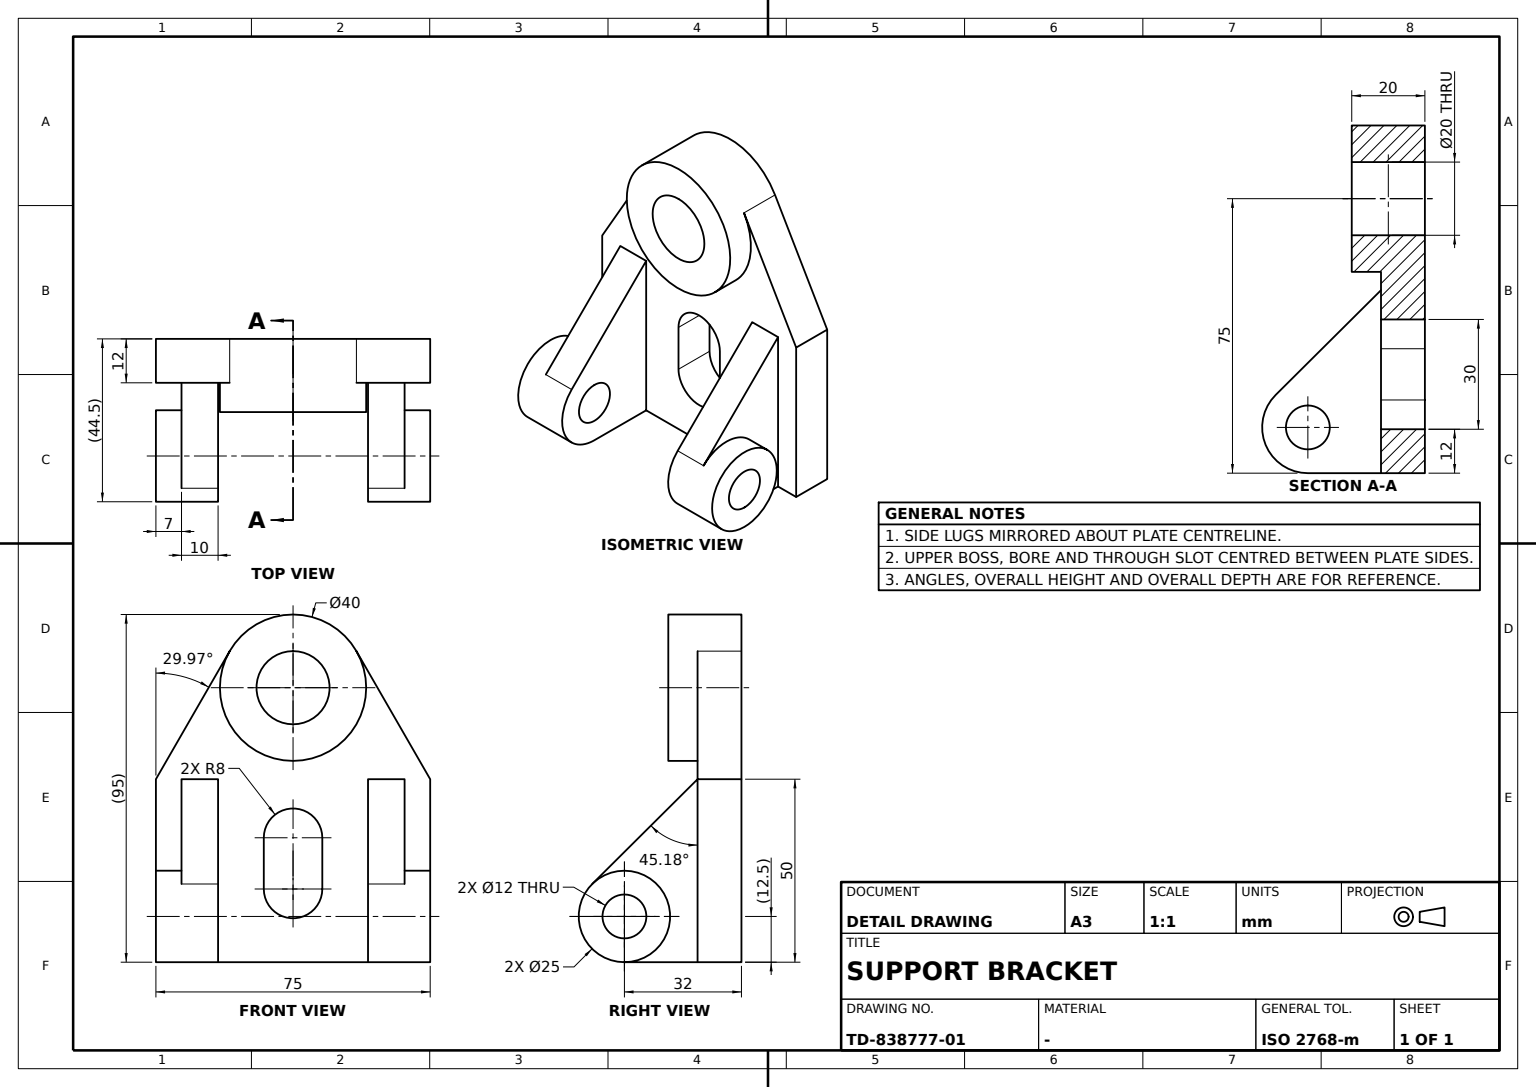
ISO-10303-21;
HEADER;
FILE_DESCRIPTION((''),'2;1');
FILE_NAME('','',(''),(''),'','','');
FILE_SCHEMA(('AUTOMOTIVE_DESIGN'));
ENDSEC;
DATA;
#1=APPLICATION_CONTEXT('');
#2=PRODUCT_CONTEXT('',#1,'mechanical');
#3=PRODUCT('','','',(#2));
#4=PRODUCT_DEFINITION_FORMATION('','',#3);
#5=PRODUCT_DEFINITION_CONTEXT('',#1,'design');
#6=PRODUCT_DEFINITION('','',#4,#5);
#7=PRODUCT_DEFINITION_SHAPE('','',#6);
#8=(LENGTH_UNIT()NAMED_UNIT(*)SI_UNIT(.MILLI.,.METRE.));
#9=(NAMED_UNIT(*)PLANE_ANGLE_UNIT()SI_UNIT($,.RADIAN.));
#10=(NAMED_UNIT(*)SI_UNIT($,.STERADIAN.)SOLID_ANGLE_UNIT());
#11=UNCERTAINTY_MEASURE_WITH_UNIT(LENGTH_MEASURE(0.005),#8,'distance_accuracy_value','');
#12=(GEOMETRIC_REPRESENTATION_CONTEXT(3)GLOBAL_UNCERTAINTY_ASSIGNED_CONTEXT((#11))GLOBAL_UNIT_ASSIGNED_CONTEXT((#8,#9,#10))REPRESENTATION_CONTEXT('',''));
#13=CARTESIAN_POINT('',(0.,-10.,10.));
#14=VERTEX_POINT('',#13);
#15=CARTESIAN_POINT('',(0.,-10.,0.));
#16=DIRECTION('',(0.,1.,0.));
#17=DIRECTION('',(0.,0.,1.));
#18=AXIS2_PLACEMENT_3D('',#15,#16,#17);
#19=CIRCLE('',#18,10.);
#20=EDGE_CURVE('',#14,#14,#19,.T.);
#21=ORIENTED_EDGE('',*,*,#20,.F.);
#22=EDGE_LOOP('',(#21));
#23=FACE_BOUND('',#22,.T.);
#24=CARTESIAN_POINT('',(0.,10.,10.));
#25=VERTEX_POINT('',#24);
#26=CARTESIAN_POINT('',(0.,10.,0.));
#27=AXIS2_PLACEMENT_3D('',#26,#16,#17);
#28=CIRCLE('',#27,10.);
#29=EDGE_CURVE('',#25,#25,#28,.T.);
#30=ORIENTED_EDGE('',*,*,#29,.T.);
#31=EDGE_LOOP('',(#30));
#32=FACE_BOUND('',#31,.T.);
#33=CARTESIAN_POINT('',(0.,0.,0.));
#34=DIRECTION('',(-1.,0.,0.));
#35=AXIS2_PLACEMENT_3D('',#33,#16,#34);
#36=CYLINDRICAL_SURFACE('',#35,10.);
#37=ADVANCED_FACE('',(#23,#32),#36,.F.);
#38=CARTESIAN_POINT('',(-8.,-10.,-41.));
#39=VERTEX_POINT('',#38);
#40=CARTESIAN_POINT('',(8.,-10.,-41.));
#41=VERTEX_POINT('',#40);
#42=CARTESIAN_POINT('',(0.,-10.,-41.));
#43=AXIS2_PLACEMENT_3D('',#42,#16,#17);
#44=CIRCLE('',#43,8.);
#45=EDGE_CURVE('',#39,#41,#44,.T.);
#46=ORIENTED_EDGE('',*,*,#45,.F.);
#47=CARTESIAN_POINT('',(-8.,2.,-41.));
#48=VERTEX_POINT('',#47);
#49=CARTESIAN_POINT('',(-8.,-4.66,-41.));
#50=VECTOR('',#16,1000.);
#51=LINE('',#49,#50);
#52=EDGE_CURVE('',#48,#39,#51,.F.);
#53=ORIENTED_EDGE('',*,*,#52,.F.);
#54=CARTESIAN_POINT('',(8.,2.,-41.));
#55=VERTEX_POINT('',#54);
#56=CARTESIAN_POINT('',(0.,2.,-41.));
#57=DIRECTION('',(0.,-1.,0.));
#58=DIRECTION('',(0.,0.,-1.));
#59=AXIS2_PLACEMENT_3D('',#56,#57,#58);
#60=CIRCLE('',#59,8.);
#61=EDGE_CURVE('',#48,#55,#60,.F.);
#62=ORIENTED_EDGE('',*,*,#61,.T.);
#63=CARTESIAN_POINT('',(8.,-4.66,-41.));
#64=LINE('',#63,#50);
#65=EDGE_CURVE('',#55,#41,#64,.F.);
#66=ORIENTED_EDGE('',*,*,#65,.T.);
#67=EDGE_LOOP('',(#46,#53,#62,#66));
#68=FACE_BOUND('',#67,.T.);
#69=CARTESIAN_POINT('',(0.,-4.66,-41.));
#70=AXIS2_PLACEMENT_3D('',#69,#16,#34);
#71=CYLINDRICAL_SURFACE('',#70,8.);
#72=ADVANCED_FACE('',(#68),#71,.F.);
#73=CARTESIAN_POINT('',(20.5,30.811466,-53.633881));
#74=VERTEX_POINT('',#73);
#75=CARTESIAN_POINT('',(20.5,22.,-75.));
#76=VERTEX_POINT('',#75);
#77=CARTESIAN_POINT('',(20.5,22.,-62.5));
#78=AXIS2_PLACEMENT_3D('',#77,#34,#17);
#79=CIRCLE('',#78,12.5);
#80=EDGE_CURVE('',#74,#76,#79,.T.);
#81=ORIENTED_EDGE('',*,*,#80,.T.);
#82=CARTESIAN_POINT('',(20.5,2.,-75.));
#83=VERTEX_POINT('',#82);
#84=CARTESIAN_POINT('',(20.5,0.,-75.));
#85=LINE('',#84,#50);
#86=EDGE_CURVE('',#83,#76,#85,.T.);
#87=ORIENTED_EDGE('',*,*,#86,.F.);
#88=CARTESIAN_POINT('',(20.5,2.,-25.));
#89=VERTEX_POINT('',#88);
#90=CARTESIAN_POINT('',(20.5,2.,0.));
#91=VECTOR('',#58,1000.);
#92=LINE('',#90,#91);
#93=EDGE_CURVE('',#89,#83,#92,.T.);
#94=ORIENTED_EDGE('',*,*,#93,.F.);
#95=CARTESIAN_POINT('',(20.5,-11.505944,-11.577303));
#96=DIRECTION('',(0.,-0.709289323,0.704917481));
#97=VECTOR('',#96,1000.);
#98=LINE('',#95,#97);
#99=EDGE_CURVE('',#74,#89,#98,.T.);
#100=ORIENTED_EDGE('',*,*,#99,.F.);
#101=EDGE_LOOP('',(#81,#87,#94,#100));
#102=FACE_BOUND('',#101,.T.);
#103=CARTESIAN_POINT('',(20.5,22.,-56.5));
#104=VERTEX_POINT('',#103);
#105=CIRCLE('',#78,6.);
#106=EDGE_CURVE('',#104,#104,#105,.T.);
#107=ORIENTED_EDGE('',*,*,#106,.F.);
#108=EDGE_LOOP('',(#107));
#109=FACE_BOUND('',#108,.T.);
#110=CARTESIAN_POINT('',(20.5,0.,0.));
#111=AXIS2_PLACEMENT_3D('',#110,#34,#57);
#112=PLANE('',#111);
#113=ADVANCED_FACE('',(#102,#109),#112,.T.);
#114=CARTESIAN_POINT('',(17.326458,-10.,9.989687));
#115=VERTEX_POINT('',#114);
#116=CARTESIAN_POINT('',(17.326458,2.,9.989687));
#117=VERTEX_POINT('',#116);
#118=CARTESIAN_POINT('',(17.326458,0.,9.989687));
#119=LINE('',#118,#50);
#120=EDGE_CURVE('',#115,#117,#119,.T.);
#121=ORIENTED_EDGE('',*,*,#120,.F.);
#122=CARTESIAN_POINT('',(37.5,-10.,-25.));
#123=VERTEX_POINT('',#122);
#124=DIRECTION('',(-0.499484358,0.,0.866322905));
#125=VECTOR('',#124,1000.);
#126=LINE('',#114,#125);
#127=EDGE_CURVE('',#123,#115,#126,.T.);
#128=ORIENTED_EDGE('',*,*,#127,.F.);
#129=CARTESIAN_POINT('',(37.5,2.,-25.));
#130=VERTEX_POINT('',#129);
#131=LINE('',#122,#50);
#132=EDGE_CURVE('',#123,#130,#131,.T.);
#133=ORIENTED_EDGE('',*,*,#132,.T.);
#134=LINE('',#129,#125);
#135=EDGE_CURVE('',#130,#117,#134,.T.);
#136=ORIENTED_EDGE('',*,*,#135,.T.);
#137=EDGE_LOOP('',(#121,#128,#133,#136));
#138=FACE_BOUND('',#137,.T.);
#139=DIRECTION('',(-0.866322905,0.,-0.499484358));
#140=AXIS2_PLACEMENT_3D('',#122,#139,#124);
#141=PLANE('',#140);
#142=ADVANCED_FACE('',(#138),#141,.F.);
#143=CARTESIAN_POINT('',(30.5,2.,-75.));
#144=VERTEX_POINT('',#143);
#145=CARTESIAN_POINT('',(30.5,22.,-75.));
#146=VERTEX_POINT('',#145);
#147=CARTESIAN_POINT('',(30.5,0.,-75.));
#148=LINE('',#147,#50);
#149=EDGE_CURVE('',#144,#146,#148,.T.);
#150=ORIENTED_EDGE('',*,*,#149,.T.);
#151=CARTESIAN_POINT('',(30.5,30.811468,-53.633883));
#152=VERTEX_POINT('',#151);
#153=CARTESIAN_POINT('',(30.5,22.,-62.5));
#154=AXIS2_PLACEMENT_3D('',#153,#34,#17);
#155=CIRCLE('',#154,12.5);
#156=EDGE_CURVE('',#146,#152,#155,.T.);
#157=ORIENTED_EDGE('',*,*,#156,.T.);
#158=CARTESIAN_POINT('',(30.5,2.,-25.));
#159=VERTEX_POINT('',#158);
#160=CARTESIAN_POINT('',(30.5,-11.505944,-11.577303));
#161=LINE('',#160,#97);
#162=EDGE_CURVE('',#152,#159,#161,.T.);
#163=ORIENTED_EDGE('',*,*,#162,.T.);
#164=CARTESIAN_POINT('',(30.5,2.,0.));
#165=LINE('',#164,#91);
#166=EDGE_CURVE('',#159,#144,#165,.T.);
#167=ORIENTED_EDGE('',*,*,#166,.T.);
#168=EDGE_LOOP('',(#150,#157,#163,#167));
#169=FACE_BOUND('',#168,.T.);
#170=CARTESIAN_POINT('',(30.5,0.,0.));
#171=AXIS2_PLACEMENT_3D('',#170,#34,#57);
#172=PLANE('',#171);
#173=ADVANCED_FACE('',(#169),#172,.F.);
#174=CARTESIAN_POINT('',(37.5,2.,-75.));
#175=VERTEX_POINT('',#174);
#176=VECTOR('',#17,1000.);
#177=LINE('',#174,#176);
#178=EDGE_CURVE('',#175,#130,#177,.T.);
#179=ORIENTED_EDGE('',*,*,#178,.T.);
#180=ORIENTED_EDGE('',*,*,#132,.F.);
#181=CARTESIAN_POINT('',(37.5,-10.,-75.));
#182=VERTEX_POINT('',#181);
#183=CARTESIAN_POINT('',(37.5,-10.,0.));
#184=LINE('',#183,#176);
#185=EDGE_CURVE('',#182,#123,#184,.T.);
#186=ORIENTED_EDGE('',*,*,#185,.F.);
#187=LINE('',#181,#50);
#188=EDGE_CURVE('',#182,#175,#187,.T.);
#189=ORIENTED_EDGE('',*,*,#188,.T.);
#190=EDGE_LOOP('',(#179,#180,#186,#189));
#191=FACE_BOUND('',#190,.T.);
#192=AXIS2_PLACEMENT_3D('',#181,#34,#17);
#193=PLANE('',#192);
#194=ADVANCED_FACE('',(#191),#193,.F.);
#195=CARTESIAN_POINT('',(37.5,22.,-50.));
#196=VERTEX_POINT('',#195);
#197=CARTESIAN_POINT('',(37.5,22.,-62.5));
#198=AXIS2_PLACEMENT_3D('',#197,#34,#17);
#199=CIRCLE('',#198,12.5);
#200=EDGE_CURVE('',#196,#196,#199,.F.);
#201=ORIENTED_EDGE('',*,*,#200,.F.);
#202=EDGE_LOOP('',(#201));
#203=FACE_BOUND('',#202,.T.);
#204=CARTESIAN_POINT('',(31.5,22.,-75.));
#205=DIRECTION('',(1.,0.,0.));
#206=VECTOR('',#205,1000.);
#207=LINE('',#204,#206);
#208=EDGE_CURVE('',#146,#76,#207,.F.);
#209=ORIENTED_EDGE('',*,*,#208,.T.);
#210=ORIENTED_EDGE('',*,*,#80,.F.);
#211=CARTESIAN_POINT('',(31.5,30.811469,-53.633883));
#212=LINE('',#211,#206);
#213=EDGE_CURVE('',#152,#74,#212,.F.);
#214=ORIENTED_EDGE('',*,*,#213,.F.);
#215=ORIENTED_EDGE('',*,*,#156,.F.);
#216=EDGE_LOOP('',(#209,#210,#214,#215));
#217=FACE_BOUND('',#216,.T.);
#218=CARTESIAN_POINT('',(31.5,22.,-62.5));
#219=AXIS2_PLACEMENT_3D('',#218,#205,#16);
#220=CYLINDRICAL_SURFACE('',#219,12.5);
#221=ADVANCED_FACE('',(#203,#217),#220,.T.);
#222=CARTESIAN_POINT('',(-30.5,2.,-25.));
#223=VERTEX_POINT('',#222);
#224=CARTESIAN_POINT('',(-20.5,2.,-25.));
#225=VERTEX_POINT('',#224);
#226=CARTESIAN_POINT('',(0.,2.,-25.));
#227=LINE('',#226,#206);
#228=EDGE_CURVE('',#223,#225,#227,.T.);
#229=ORIENTED_EDGE('',*,*,#228,.T.);
#230=CARTESIAN_POINT('',(-20.5,30.811469,-53.633883));
#231=VERTEX_POINT('',#230);
#232=CARTESIAN_POINT('',(-20.5,-11.505944,-11.577303));
#233=LINE('',#232,#97);
#234=EDGE_CURVE('',#231,#225,#233,.T.);
#235=ORIENTED_EDGE('',*,*,#234,.F.);
#236=CARTESIAN_POINT('',(-30.5,30.811469,-53.633883));
#237=VERTEX_POINT('',#236);
#238=EDGE_CURVE('',#237,#231,#212,.T.);
#239=ORIENTED_EDGE('',*,*,#238,.F.);
#240=CARTESIAN_POINT('',(-30.5,-11.505944,-11.577303));
#241=LINE('',#240,#97);
#242=EDGE_CURVE('',#237,#223,#241,.T.);
#243=ORIENTED_EDGE('',*,*,#242,.T.);
#244=EDGE_LOOP('',(#229,#235,#239,#243));
#245=FACE_BOUND('',#244,.T.);
#246=CARTESIAN_POINT('',(25.5,30.811469,-53.633883));
#247=DIRECTION('',(0.,-0.704917481,-0.709289323));
#248=AXIS2_PLACEMENT_3D('',#246,#247,#96);
#249=PLANE('',#248);
#250=ADVANCED_FACE('',(#245),#249,.F.);
#251=CARTESIAN_POINT('',(-17.326458,2.,9.989687));
#252=VERTEX_POINT('',#251);
#253=CARTESIAN_POINT('',(-37.5,2.,-25.));
#254=VERTEX_POINT('',#253);
#255=DIRECTION('',(-0.499484358,0.,-0.866322905));
#256=VECTOR('',#255,1000.);
#257=LINE('',#251,#256);
#258=EDGE_CURVE('',#252,#254,#257,.T.);
#259=ORIENTED_EDGE('',*,*,#258,.T.);
#260=CARTESIAN_POINT('',(-37.5,-10.,-25.));
#261=VERTEX_POINT('',#260);
#262=LINE('',#260,#50);
#263=EDGE_CURVE('',#261,#254,#262,.T.);
#264=ORIENTED_EDGE('',*,*,#263,.F.);
#265=CARTESIAN_POINT('',(-17.326458,-10.,9.989687));
#266=VERTEX_POINT('',#265);
#267=LINE('',#265,#256);
#268=EDGE_CURVE('',#266,#261,#267,.T.);
#269=ORIENTED_EDGE('',*,*,#268,.F.);
#270=CARTESIAN_POINT('',(-17.326458,0.,9.989687));
#271=LINE('',#270,#50);
#272=EDGE_CURVE('',#266,#252,#271,.T.);
#273=ORIENTED_EDGE('',*,*,#272,.T.);
#274=EDGE_LOOP('',(#259,#264,#269,#273));
#275=FACE_BOUND('',#274,.T.);
#276=DIRECTION('',(0.866322905,0.,-0.499484358));
#277=AXIS2_PLACEMENT_3D('',#265,#276,#255);
#278=PLANE('',#277);
#279=ADVANCED_FACE('',(#275),#278,.F.);
#280=CARTESIAN_POINT('',(-37.5,22.,-75.));
#281=VERTEX_POINT('',#280);
#282=CARTESIAN_POINT('',(-37.5,22.,-62.5));
#283=AXIS2_PLACEMENT_3D('',#282,#205,#58);
#284=CIRCLE('',#283,12.5);
#285=EDGE_CURVE('',#281,#281,#284,.T.);
#286=ORIENTED_EDGE('',*,*,#285,.F.);
#287=EDGE_LOOP('',(#286));
#288=FACE_BOUND('',#287,.T.);
#289=CARTESIAN_POINT('',(-37.5,22.,-68.5));
#290=VERTEX_POINT('',#289);
#291=CIRCLE('',#283,6.);
#292=EDGE_CURVE('',#290,#290,#291,.T.);
#293=ORIENTED_EDGE('',*,*,#292,.T.);
#294=EDGE_LOOP('',(#293));
#295=FACE_BOUND('',#294,.T.);
#296=AXIS2_PLACEMENT_3D('',#260,#205,#58);
#297=PLANE('',#296);
#298=ADVANCED_FACE('',(#288,#295),#297,.F.);
#299=ORIENTED_EDGE('',*,*,#234,.T.);
#300=CARTESIAN_POINT('',(-20.5,2.,-75.));
#301=VERTEX_POINT('',#300);
#302=CARTESIAN_POINT('',(-20.5,2.,0.));
#303=LINE('',#302,#91);
#304=EDGE_CURVE('',#225,#301,#303,.T.);
#305=ORIENTED_EDGE('',*,*,#304,.T.);
#306=CARTESIAN_POINT('',(-20.5,21.999997,-75.));
#307=VERTEX_POINT('',#306);
#308=CARTESIAN_POINT('',(-20.5,0.,-75.));
#309=LINE('',#308,#50);
#310=EDGE_CURVE('',#301,#307,#309,.T.);
#311=ORIENTED_EDGE('',*,*,#310,.T.);
#312=CARTESIAN_POINT('',(-20.5,22.,-62.5));
#313=AXIS2_PLACEMENT_3D('',#312,#34,#17);
#314=CIRCLE('',#313,12.5);
#315=EDGE_CURVE('',#231,#307,#314,.T.);
#316=ORIENTED_EDGE('',*,*,#315,.F.);
#317=EDGE_LOOP('',(#299,#305,#311,#316));
#318=FACE_BOUND('',#317,.T.);
#319=CARTESIAN_POINT('',(-20.5,22.,-56.5));
#320=VERTEX_POINT('',#319);
#321=CIRCLE('',#313,6.);
#322=EDGE_CURVE('',#320,#320,#321,.T.);
#323=ORIENTED_EDGE('',*,*,#322,.T.);
#324=EDGE_LOOP('',(#323));
#325=FACE_BOUND('',#324,.T.);
#326=CARTESIAN_POINT('',(-20.5,0.,0.));
#327=AXIS2_PLACEMENT_3D('',#326,#34,#57);
#328=PLANE('',#327);
#329=ADVANCED_FACE('',(#318,#325),#328,.F.);
#330=ORIENTED_EDGE('',*,*,#263,.T.);
#331=CARTESIAN_POINT('',(-37.5,2.,-75.));
#332=VERTEX_POINT('',#331);
#333=LINE('',#253,#91);
#334=EDGE_CURVE('',#254,#332,#333,.T.);
#335=ORIENTED_EDGE('',*,*,#334,.T.);
#336=CARTESIAN_POINT('',(-37.5,-10.,-75.));
#337=VERTEX_POINT('',#336);
#338=LINE('',#336,#50);
#339=EDGE_CURVE('',#337,#332,#338,.T.);
#340=ORIENTED_EDGE('',*,*,#339,.F.);
#341=CARTESIAN_POINT('',(-37.5,-10.,0.));
#342=LINE('',#341,#91);
#343=EDGE_CURVE('',#261,#337,#342,.T.);
#344=ORIENTED_EDGE('',*,*,#343,.F.);
#345=EDGE_LOOP('',(#330,#335,#340,#344));
#346=FACE_BOUND('',#345,.T.);
#347=ADVANCED_FACE('',(#346),#297,.F.);
#348=ORIENTED_EDGE('',*,*,#292,.F.);
#349=EDGE_LOOP('',(#348));
#350=FACE_BOUND('',#349,.T.);
#351=ORIENTED_EDGE('',*,*,#322,.F.);
#352=EDGE_LOOP('',(#351));
#353=FACE_BOUND('',#352,.T.);
#354=CYLINDRICAL_SURFACE('',#219,6.);
#355=ADVANCED_FACE('',(#350,#353),#354,.F.);
#356=CARTESIAN_POINT('',(0.,-10.,-75.));
#357=LINE('',#356,#206);
#358=EDGE_CURVE('',#337,#182,#357,.T.);
#359=ORIENTED_EDGE('',*,*,#358,.F.);
#360=ORIENTED_EDGE('',*,*,#339,.T.);
#361=CARTESIAN_POINT('',(-30.5,2.,-75.));
#362=VERTEX_POINT('',#361);
#363=LINE('',#331,#206);
#364=EDGE_CURVE('',#332,#362,#363,.T.);
#365=ORIENTED_EDGE('',*,*,#364,.T.);
#366=CARTESIAN_POINT('',(-30.5,22.,-75.));
#367=VERTEX_POINT('',#366);
#368=CARTESIAN_POINT('',(-30.5,0.,-75.));
#369=LINE('',#368,#50);
#370=EDGE_CURVE('',#362,#367,#369,.T.);
#371=ORIENTED_EDGE('',*,*,#370,.T.);
#372=EDGE_CURVE('',#367,#307,#207,.T.);
#373=ORIENTED_EDGE('',*,*,#372,.T.);
#374=ORIENTED_EDGE('',*,*,#310,.F.);
#375=EDGE_CURVE('',#301,#83,#363,.T.);
#376=ORIENTED_EDGE('',*,*,#375,.T.);
#377=ORIENTED_EDGE('',*,*,#86,.T.);
#378=ORIENTED_EDGE('',*,*,#208,.F.);
#379=ORIENTED_EDGE('',*,*,#149,.F.);
#380=EDGE_CURVE('',#144,#175,#363,.T.);
#381=ORIENTED_EDGE('',*,*,#380,.T.);
#382=ORIENTED_EDGE('',*,*,#188,.F.);
#383=EDGE_LOOP('',(#359,#360,#365,#371,#373,#374,#376,#377,#378,#379,#381,#382));
#384=FACE_BOUND('',#383,.T.);
#385=AXIS2_PLACEMENT_3D('',#336,#17,#205);
#386=PLANE('',#385);
#387=ADVANCED_FACE('',(#384),#386,.F.);
#388=ORIENTED_EDGE('',*,*,#99,.T.);
#389=CARTESIAN_POINT('',(25.5,2.,-25.));
#390=VECTOR('',#34,1000.);
#391=LINE('',#389,#390);
#392=EDGE_CURVE('',#159,#89,#391,.T.);
#393=ORIENTED_EDGE('',*,*,#392,.F.);
#394=ORIENTED_EDGE('',*,*,#162,.F.);
#395=ORIENTED_EDGE('',*,*,#213,.T.);
#396=EDGE_LOOP('',(#388,#393,#394,#395));
#397=FACE_BOUND('',#396,.T.);
#398=ADVANCED_FACE('',(#397),#249,.F.);
#399=ORIENTED_EDGE('',*,*,#65,.F.);
#400=CARTESIAN_POINT('',(8.,2.,-55.));
#401=VERTEX_POINT('',#400);
#402=CARTESIAN_POINT('',(8.,2.,0.));
#403=LINE('',#402,#91);
#404=EDGE_CURVE('',#55,#401,#403,.T.);
#405=ORIENTED_EDGE('',*,*,#404,.T.);
#406=CARTESIAN_POINT('',(8.,-10.,-55.));
#407=VERTEX_POINT('',#406);
#408=CARTESIAN_POINT('',(8.,-4.66,-55.));
#409=LINE('',#408,#50);
#410=EDGE_CURVE('',#401,#407,#409,.F.);
#411=ORIENTED_EDGE('',*,*,#410,.T.);
#412=LINE('',#40,#91);
#413=EDGE_CURVE('',#41,#407,#412,.T.);
#414=ORIENTED_EDGE('',*,*,#413,.F.);
#415=EDGE_LOOP('',(#399,#405,#411,#414));
#416=FACE_BOUND('',#415,.T.);
#417=AXIS2_PLACEMENT_3D('',#54,#34,#58);
#418=PLANE('',#417);
#419=ADVANCED_FACE('',(#416),#418,.T.);
#420=ORIENTED_EDGE('',*,*,#392,.T.);
#421=ORIENTED_EDGE('',*,*,#93,.T.);
#422=ORIENTED_EDGE('',*,*,#375,.F.);
#423=ORIENTED_EDGE('',*,*,#304,.F.);
#424=ORIENTED_EDGE('',*,*,#228,.F.);
#425=CARTESIAN_POINT('',(-30.5,2.,0.));
#426=LINE('',#425,#91);
#427=EDGE_CURVE('',#223,#362,#426,.T.);
#428=ORIENTED_EDGE('',*,*,#427,.T.);
#429=ORIENTED_EDGE('',*,*,#364,.F.);
#430=ORIENTED_EDGE('',*,*,#334,.F.);
#431=ORIENTED_EDGE('',*,*,#258,.F.);
#432=CARTESIAN_POINT('',(0.,2.,0.));
#433=AXIS2_PLACEMENT_3D('',#432,#57,#58);
#434=CIRCLE('',#433,20.);
#435=EDGE_CURVE('',#252,#117,#434,.T.);
#436=ORIENTED_EDGE('',*,*,#435,.T.);
#437=ORIENTED_EDGE('',*,*,#135,.F.);
#438=ORIENTED_EDGE('',*,*,#178,.F.);
#439=ORIENTED_EDGE('',*,*,#380,.F.);
#440=ORIENTED_EDGE('',*,*,#166,.F.);
#441=EDGE_LOOP('',(#420,#421,#422,#423,#424,#428,#429,#430,#431,#436,#437,#438,#439,#440));
#442=FACE_BOUND('',#441,.T.);
#443=CARTESIAN_POINT('',(-8.,2.,-55.));
#444=VERTEX_POINT('',#443);
#445=CARTESIAN_POINT('',(0.,2.,-55.));
#446=AXIS2_PLACEMENT_3D('',#445,#57,#58);
#447=CIRCLE('',#446,8.);
#448=EDGE_CURVE('',#401,#444,#447,.F.);
#449=ORIENTED_EDGE('',*,*,#448,.F.);
#450=ORIENTED_EDGE('',*,*,#404,.F.);
#451=ORIENTED_EDGE('',*,*,#61,.F.);
#452=CARTESIAN_POINT('',(-8.,2.,0.));
#453=LINE('',#452,#91);
#454=EDGE_CURVE('',#48,#444,#453,.T.);
#455=ORIENTED_EDGE('',*,*,#454,.T.);
#456=EDGE_LOOP('',(#449,#450,#451,#455));
#457=FACE_BOUND('',#456,.T.);
#458=AXIS2_PLACEMENT_3D('',#432,#57,#205);
#459=PLANE('',#458);
#460=ADVANCED_FACE('',(#442,#457),#459,.F.);
#461=CARTESIAN_POINT('',(-30.5,22.,-62.5));
#462=AXIS2_PLACEMENT_3D('',#461,#34,#17);
#463=CIRCLE('',#462,12.5);
#464=EDGE_CURVE('',#367,#237,#463,.T.);
#465=ORIENTED_EDGE('',*,*,#464,.F.);
#466=ORIENTED_EDGE('',*,*,#370,.F.);
#467=ORIENTED_EDGE('',*,*,#427,.F.);
#468=ORIENTED_EDGE('',*,*,#242,.F.);
#469=EDGE_LOOP('',(#465,#466,#467,#468));
#470=FACE_BOUND('',#469,.T.);
#471=CARTESIAN_POINT('',(-30.5,0.,0.));
#472=AXIS2_PLACEMENT_3D('',#471,#34,#57);
#473=PLANE('',#472);
#474=ADVANCED_FACE('',(#470),#473,.T.);
#475=ORIENTED_EDGE('',*,*,#464,.T.);
#476=ORIENTED_EDGE('',*,*,#238,.T.);
#477=ORIENTED_EDGE('',*,*,#315,.T.);
#478=ORIENTED_EDGE('',*,*,#372,.F.);
#479=EDGE_LOOP('',(#475,#476,#477,#478));
#480=FACE_BOUND('',#479,.T.);
#481=ORIENTED_EDGE('',*,*,#285,.T.);
#482=EDGE_LOOP('',(#481));
#483=FACE_BOUND('',#482,.T.);
#484=ADVANCED_FACE('',(#480,#483),#220,.T.);
#485=CARTESIAN_POINT('',(0.,10.,20.));
#486=VERTEX_POINT('',#485);
#487=CIRCLE('',#27,20.);
#488=EDGE_CURVE('',#486,#486,#487,.T.);
#489=ORIENTED_EDGE('',*,*,#488,.T.);
#490=EDGE_LOOP('',(#489));
#491=FACE_BOUND('',#490,.T.);
#492=ORIENTED_EDGE('',*,*,#29,.F.);
#493=EDGE_LOOP('',(#492));
#494=FACE_BOUND('',#493,.T.);
#495=AXIS2_PLACEMENT_3D('',#26,#16,#34);
#496=PLANE('',#495);
#497=ADVANCED_FACE('',(#491,#494),#496,.T.);
#498=ORIENTED_EDGE('',*,*,#106,.T.);
#499=EDGE_LOOP('',(#498));
#500=FACE_BOUND('',#499,.T.);
#501=CARTESIAN_POINT('',(37.5,22.,-56.5));
#502=VERTEX_POINT('',#501);
#503=CIRCLE('',#198,6.);
#504=EDGE_CURVE('',#502,#502,#503,.F.);
#505=ORIENTED_EDGE('',*,*,#504,.T.);
#506=EDGE_LOOP('',(#505));
#507=FACE_BOUND('',#506,.T.);
#508=ADVANCED_FACE('',(#500,#507),#354,.F.);
#509=CIRCLE('',#18,20.);
#510=EDGE_CURVE('',#266,#115,#509,.T.);
#511=ORIENTED_EDGE('',*,*,#510,.F.);
#512=ORIENTED_EDGE('',*,*,#268,.T.);
#513=ORIENTED_EDGE('',*,*,#343,.T.);
#514=ORIENTED_EDGE('',*,*,#358,.T.);
#515=ORIENTED_EDGE('',*,*,#185,.T.);
#516=ORIENTED_EDGE('',*,*,#127,.T.);
#517=EDGE_LOOP('',(#511,#512,#513,#514,#515,#516));
#518=FACE_BOUND('',#517,.T.);
#519=ORIENTED_EDGE('',*,*,#20,.T.);
#520=EDGE_LOOP('',(#519));
#521=FACE_BOUND('',#520,.T.);
#522=CARTESIAN_POINT('',(-8.,-10.,-55.));
#523=VERTEX_POINT('',#522);
#524=CARTESIAN_POINT('',(0.,-10.,-55.));
#525=AXIS2_PLACEMENT_3D('',#524,#16,#17);
#526=CIRCLE('',#525,8.);
#527=EDGE_CURVE('',#407,#523,#526,.T.);
#528=ORIENTED_EDGE('',*,*,#527,.T.);
#529=LINE('',#38,#91);
#530=EDGE_CURVE('',#39,#523,#529,.T.);
#531=ORIENTED_EDGE('',*,*,#530,.F.);
#532=ORIENTED_EDGE('',*,*,#45,.T.);
#533=ORIENTED_EDGE('',*,*,#413,.T.);
#534=EDGE_LOOP('',(#528,#531,#532,#533));
#535=FACE_BOUND('',#534,.T.);
#536=AXIS2_PLACEMENT_3D('',#15,#16,#34);
#537=PLANE('',#536);
#538=ADVANCED_FACE('',(#518,#521,#535),#537,.F.);
#539=ORIENTED_EDGE('',*,*,#527,.F.);
#540=ORIENTED_EDGE('',*,*,#410,.F.);
#541=ORIENTED_EDGE('',*,*,#448,.T.);
#542=CARTESIAN_POINT('',(-8.,-4.66,-55.));
#543=LINE('',#542,#50);
#544=EDGE_CURVE('',#444,#523,#543,.F.);
#545=ORIENTED_EDGE('',*,*,#544,.T.);
#546=EDGE_LOOP('',(#539,#540,#541,#545));
#547=FACE_BOUND('',#546,.T.);
#548=CARTESIAN_POINT('',(0.,-4.66,-55.));
#549=AXIS2_PLACEMENT_3D('',#548,#16,#34);
#550=CYLINDRICAL_SURFACE('',#549,8.);
#551=ADVANCED_FACE('',(#547),#550,.F.);
#552=ORIENTED_EDGE('',*,*,#200,.T.);
#553=EDGE_LOOP('',(#552));
#554=FACE_BOUND('',#553,.T.);
#555=ORIENTED_EDGE('',*,*,#504,.F.);
#556=EDGE_LOOP('',(#555));
#557=FACE_BOUND('',#556,.T.);
#558=ADVANCED_FACE('',(#554,#557),#193,.F.);
#559=ORIENTED_EDGE('',*,*,#488,.F.);
#560=EDGE_LOOP('',(#559));
#561=FACE_BOUND('',#560,.T.);
#562=ORIENTED_EDGE('',*,*,#120,.T.);
#563=ORIENTED_EDGE('',*,*,#435,.F.);
#564=ORIENTED_EDGE('',*,*,#272,.F.);
#565=ORIENTED_EDGE('',*,*,#510,.T.);
#566=EDGE_LOOP('',(#562,#563,#564,#565));
#567=FACE_BOUND('',#566,.T.);
#568=CYLINDRICAL_SURFACE('',#35,20.);
#569=ADVANCED_FACE('',(#561,#567),#568,.T.);
#570=ORIENTED_EDGE('',*,*,#52,.T.);
#571=ORIENTED_EDGE('',*,*,#530,.T.);
#572=ORIENTED_EDGE('',*,*,#544,.F.);
#573=ORIENTED_EDGE('',*,*,#454,.F.);
#574=EDGE_LOOP('',(#570,#571,#572,#573));
#575=FACE_BOUND('',#574,.T.);
#576=AXIS2_PLACEMENT_3D('',#47,#34,#58);
#577=PLANE('',#576);
#578=ADVANCED_FACE('',(#575),#577,.F.);
#579=CLOSED_SHELL('',(#37,#72,#113,#142,#173,#194,#221,#250,#279,#298,#329,#347,#355,#387,#398,#419,#460,#474,#484,#497,#508,#538,#551,#558,#569,#578));
#580=MANIFOLD_SOLID_BREP('',#579);
#581=ADVANCED_BREP_SHAPE_REPRESENTATION('',(#580),#12);
#582=SHAPE_DEFINITION_REPRESENTATION(#7,#581);
ENDSEC;
END-ISO-10303-21;
